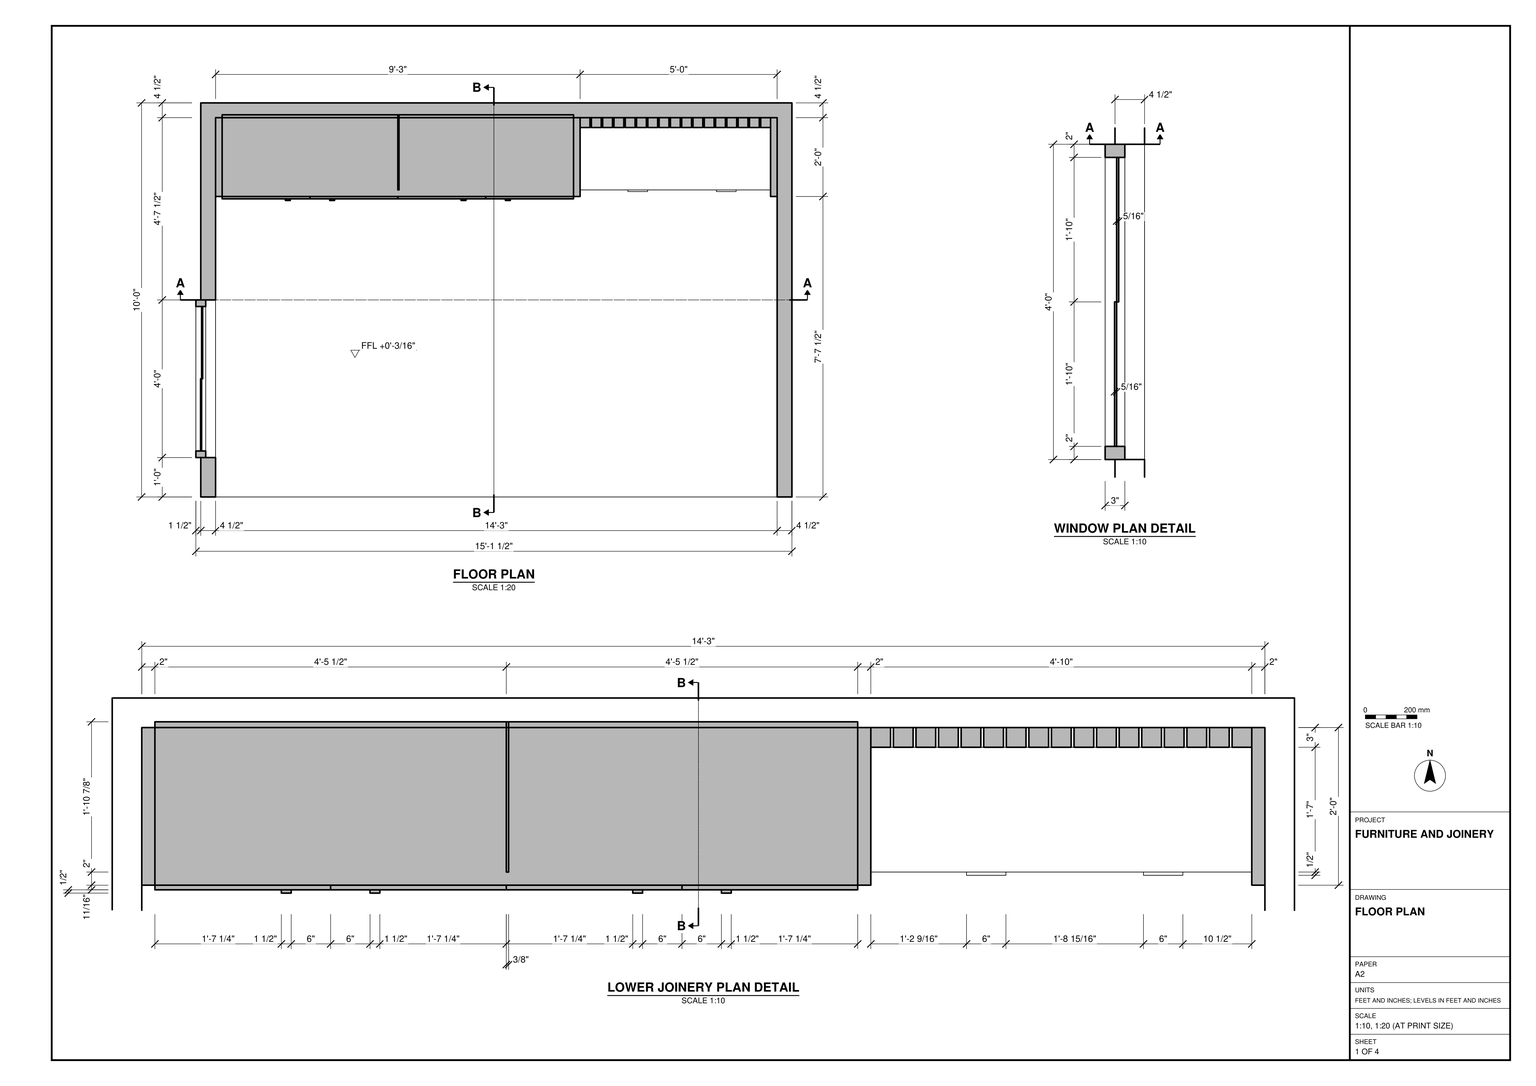
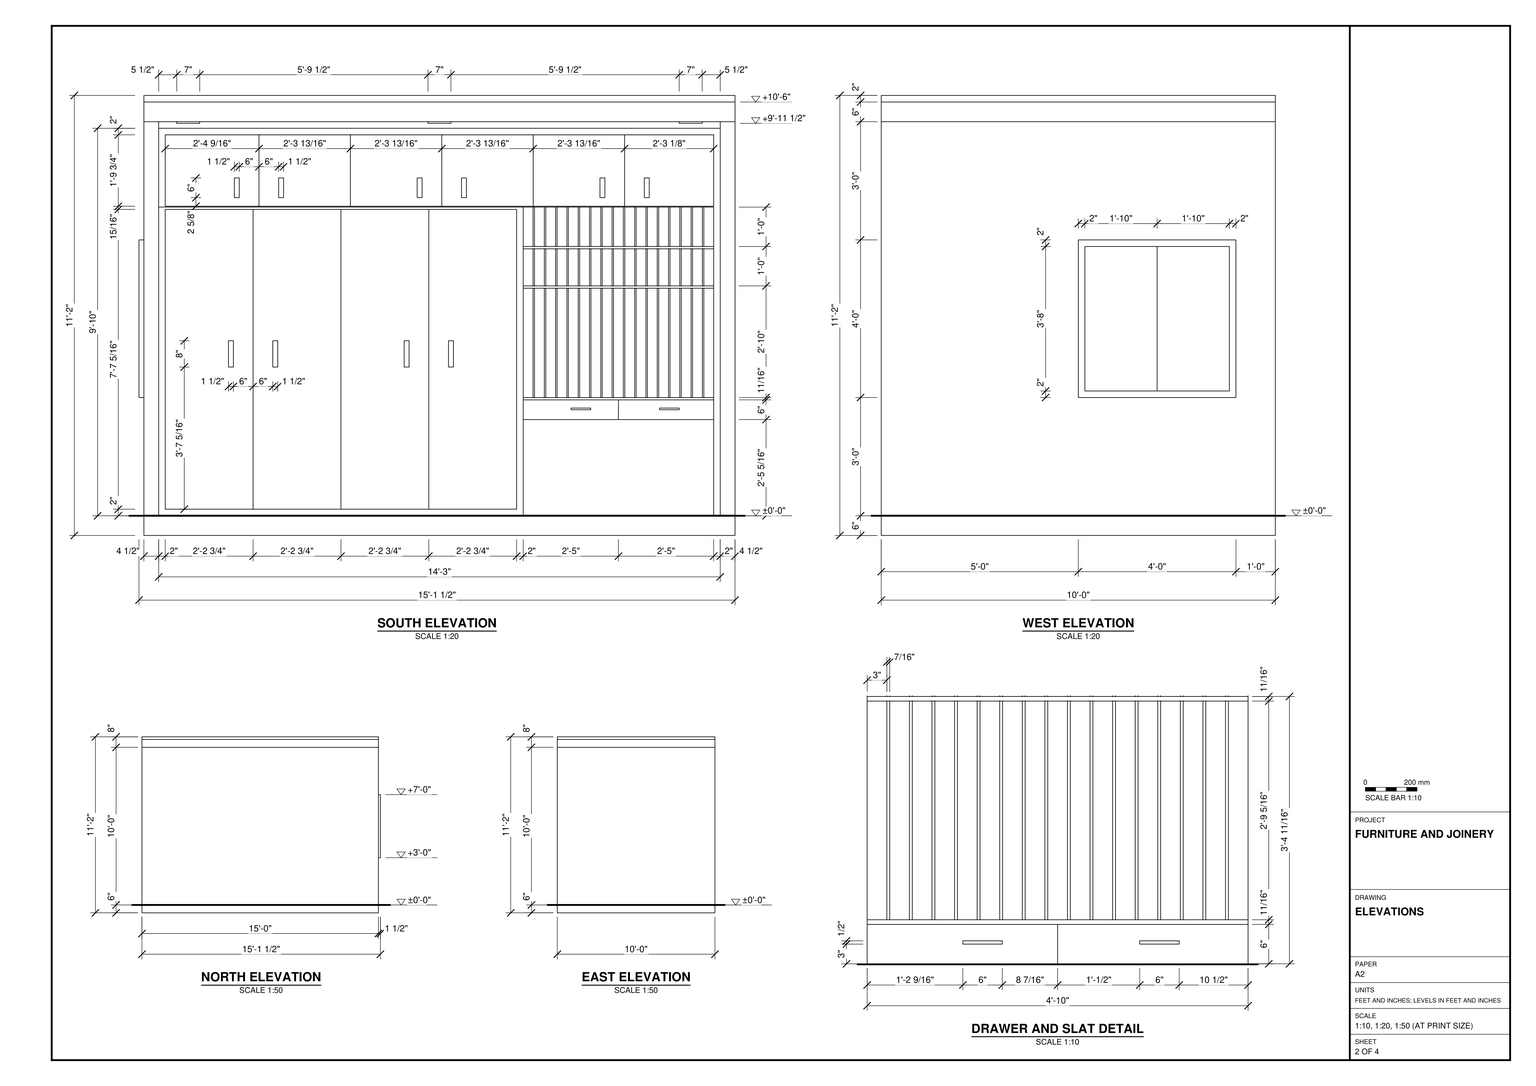
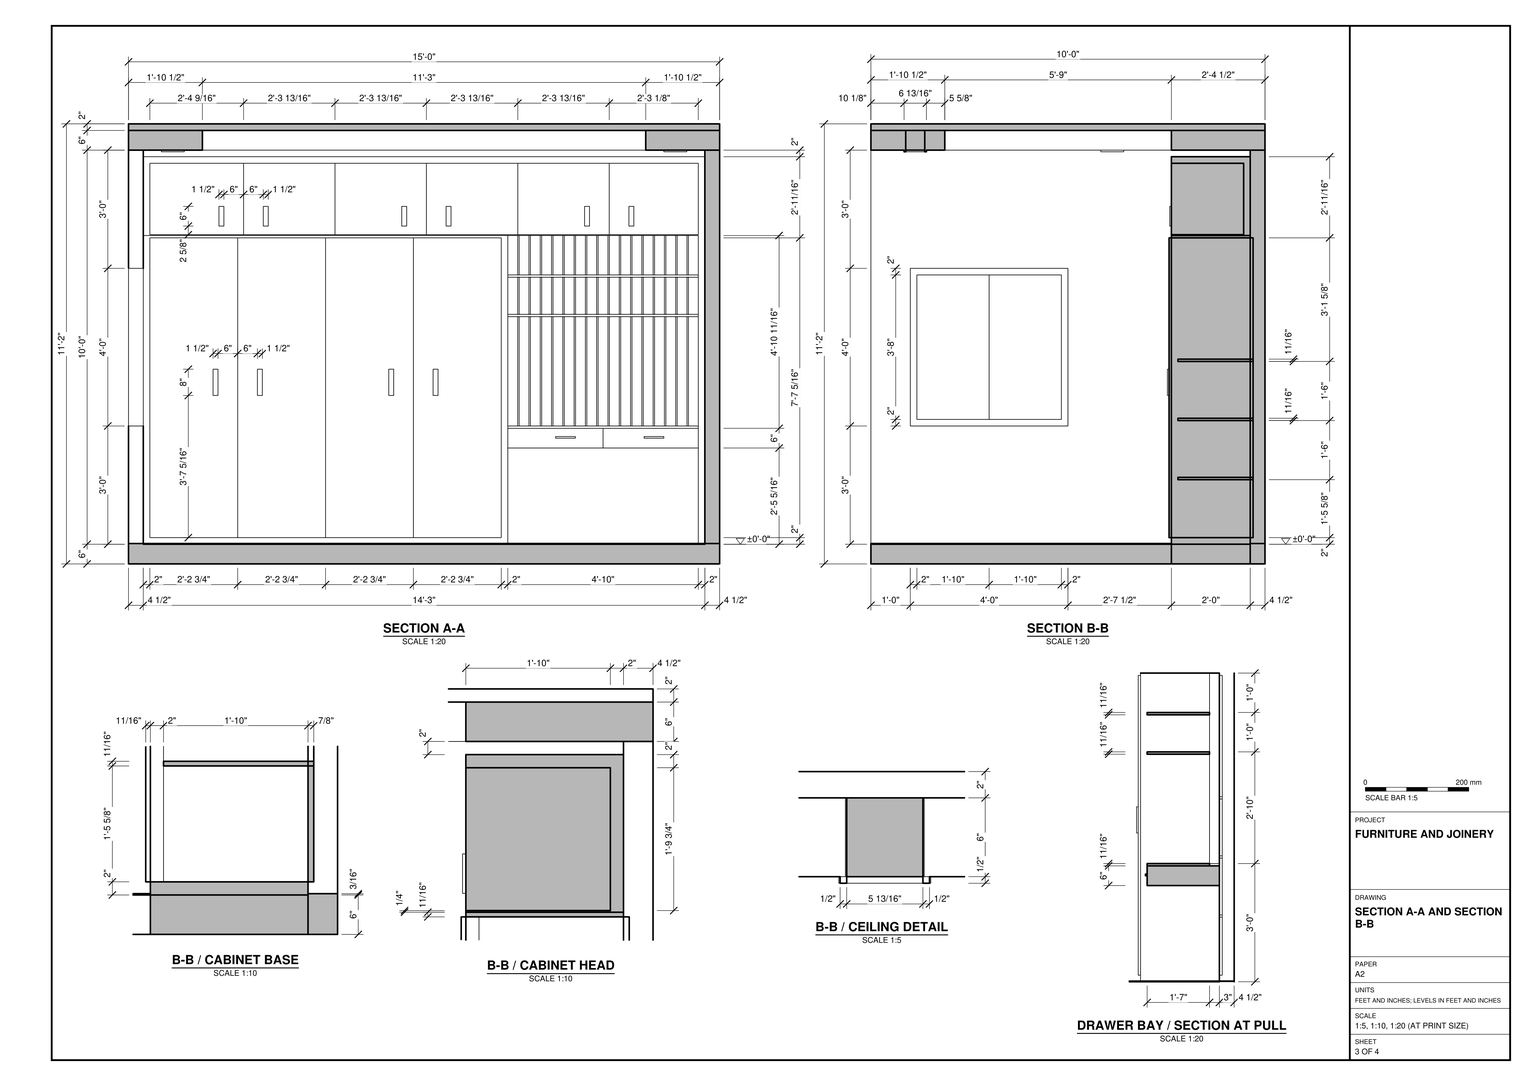
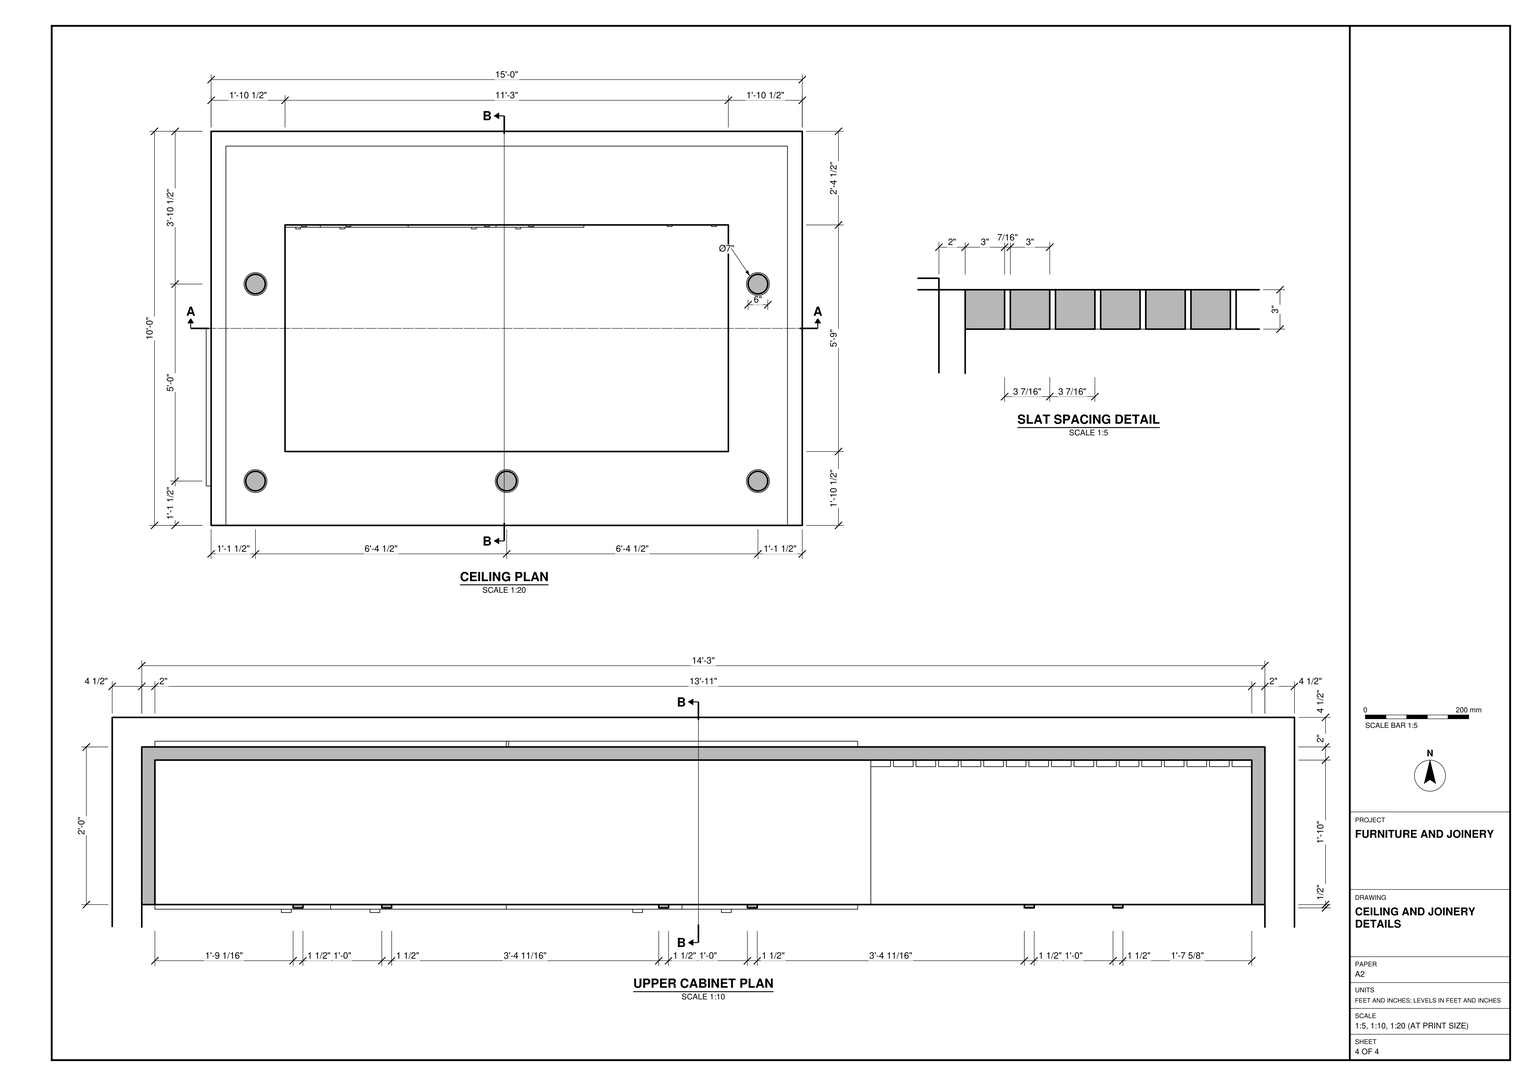
Build the wall-to-wall storage unit and its surrounding room shell in SketchUp using task_files/diagram_01.pdf. Work in feet and inches. The overall model is 15'-1 1/2" wide, 10'-0" deep and 11'-2" high. Use ±0'-0" as the ground-floor datum.

Model the floor slab, the 4 1/2" back and side walls, and the ceiling slab with its deeper perimeter section. Leave the front open as shown in plan. Fit the framed, two-panel window into the west wall at the position shown in the west elevation.

Run the joinery along the back wall. Facing the unit, place the tall wardrobe on the left, with its plinth, internal partition, shelves and paired door fronts. Continue the overhead cupboards across both the wardrobe and the open bay on the right. In that bay, model the vertical slats behind the shelves and the two shallow drawers side by side, leaving clear space beneath them. Follow the elevations for the size and orientation of the pulls.

Keep shell elements and individual joinery pieces in separate groups or components, and use components for repeated parts. Any decor or loose items may be suitable library components. Save one SketchUp model as output_files/built_in_wardrobe_with_a_slatted_drawer_bay.skp.

# SketchUp Ruby script. Lengths in inches.
U = 1.inch
M = Sketchup.active_model
def pt(a) = Geom::Point3d.new(a.map { |v| v * U })
def face(e, loops, mat)
  f = e.add_face(loops[0].map { |a| pt(a) })
  loops[1..].each { |l| e.add_face(l.map { |a| pt(a) }).erase! }
  f.material = f.back_material = mat if mat
  f
end
# faces: each face lists its corners as indices into pts; further lists are holes
def faces(e, pts, list, mat = nil) = list.each { |f| face(e, (f[0].is_a?(Array) ? f : [f]).map { |l| l.map { |i| pts[i] } }, mat) }
# xy, xz, yz: faces in a plane at the given z, y or x. An outline is a flat list of corners, or four numbers for a rectangle; further outlines are holes
def ring(l) = l.size == 4 ? [[l[0], l[1]], [l[2], l[1]], [l[2], l[3]], [l[0], l[3]]] : l.each_slice(2).to_a
def flat(e, list, mat, &to3) = list.each { |f| face(e, (f[0].is_a?(Array) ? f : [f]).map { |l| ring(l).map { |u, v| to3.(u, v) } }, mat) }
def xy(e, z, list, mat = nil) = flat(e, list, mat) { |x, y| [x, y, z] }
def xz(e, y, list, mat = nil) = flat(e, list, mat) { |x, z| [x, y, z] }
def yz(e, x, list, mat = nil) = flat(e, list, mat) { |y, z| [x, y, z] }
def lines(e, pts, list) = list.each { |a, b| e.add_line(pt(pts[a]), pt(pts[b])) }
# prism: a flat outline (further loops are holes) pulled along v
def prism(e, loops, v, mat = nil)
  f = face(e, loops, mat); d = Geom::Vector3d.new(v.map { |x| x * U })
  f.pushpull(f.normal.samedirection?(d) ? d.length : -d.length)
end
def box(e, o, s, mat = nil) = prism(e, [[o, [o[0] + s[0], o[1], o[2]], [o[0] + s[0], o[1] + s[1], o[2]], [o[0], o[1] + s[1], o[2]]]], [0, 0, s[2]], mat)
def at(x, y, z, deg = 0) = Geom::Transformation.translation(pt([x, y, z])) * Geom::Transformation.rotation(ORIGIN, Z_AXIS, deg.degrees)
def axes(o, x, y, z) = Geom::Transformation.new([*x, 0, *y, 0, *z, 0, *pt(o).to_a, 1])
def part(name) = M.definitions.add(name)
# library, detail: a bought-in or finely detailed component or shape, given as its bounding box
def library(name, o, s) = part(name).tap { |d| box(d.entities, o, s) }
def detail(e, o, s) = box(e.add_group.entities, o, s)
def put(e, d, t, mat = nil) = e.add_instance(d, t).tap { |i| i.material = mat if mat }
def group(e, t, mat = nil) = e.add_group.tap { |g| g.transformation = t; g.material = mat if mat }.entities
root = M.entities
M.materials.add("Carpaint Stochastic Gold").color = [216, 180, 130]
M.materials.add("Flooring Parquet Parallel E01 120cm").color = [119, 88, 63]
M.materials.add("Glass Yellow 001").color = [0, 0, 0]
M.materials["Glass Yellow 001"].alpha = 0.1
M.materials.add("Marble Black 100cm").color = [32, 32, 32]
M.materials.add("Metal Sandblasted Black 200cm").color = [86, 90, 95]
M.materials.add("Wood Tiles Dark Shiny 02 100cm").color = [42, 30, 20]
M.materials.add("[0023_FireBrick]").color = [236, 223, 216]
M.materials.add("[Color C06]").color = [166, 138, 92]
M.materials.add("[Color D01]").color = [255, 242, 204]
M.materials.add("[Color D05]").color = [234, 208, 139]
M.materials.add("[Color D06]").color = [170, 123, 68]
M.materials.add("[Color M00]").color = [255, 255, 255]
M.materials.add("[Color M04]").color = [142, 142, 142]
M.materials.add("[Color M06]").color = [86, 86, 86]
c1 = part("Group\#25")
box(c1.entities,[0,0,0],[0.31,22,44])
c2 = part("Group\#2")
box(c2.entities,[0,2,-0.35],[107,22.875,0.7])
p = [[24,22.5,126],[24,91.5,126],[159,91.5,126],[159,22.5,126]]
lines(root,p,[[0,1],[1,2],[2,3],[3,0]])
g1 = group(root,at(1.5,0,0))
xy(g1,0,[[4.5,0,175.5,115.5]],"[Color M04]")
xy(g1,36,[[0,12,4.5,60]],"[Color M04]")
xy(g1,84,[[0,12,4.5,60]],"[Color M04]")
xy(g1,120,[[0,0,4.5,0,4.5,115.5,175.5,115.5,175.5,0,180,0,180,120,0,120]],"[Color M04]")
xz(g1,0,[[0,0,4.5,120],[175.5,0,180,120]],"[Color M04]")
xz(g1,12,[[0,36,4.5,84]],"[Color M04]")
xz(g1,60,[[0,36,4.5,84]],"[Color M04]")
xz(g1,115.5,[[4.5,0,175.5,120]],"[Color M04]")
xz(g1,120,[[0,0,180,120]],"[Color M04]")
yz(g1,0,[[[0,0,120,120],[12,36,60,84]]],"[Color M04]")
yz(g1,4.5,[[[0,0,115.5,120],[12,36,60,84]]],"[Color M04]")
yz(g1,175.5,[[0,0,115.5,120]],"[Color M04]")
yz(g1,180,[[0,0,120,120]],"[Color M04]")
g2 = group(g1,at(0,12,36))
prism(g2,[[[-1.5,48,0],[-1.5,0,0],[-1.5,0,48],[-1.5,48,48]],[[-1.5,46,2],[-1.5,46,46],[-1.5,2,46],[-1.5,2,2]]],[3,0,0],"Metal Sandblasted Black 200cm")
put(g1,c1,at(0.25,36,38),"Glass Yellow 001")
put(g1,c1,at(-0.06,14,38),"Glass Yellow 001")
put(root,c2,at(8,91.5,20))
put(root,c2,at(8,91.5,38))
put(root,c2,at(8,91.5,56))
g3 = group(root,at(61.5,91.5,2.71))
prism(g3,[[[0,2,-0.71],[0,2,90.58],[0,24,90.58],[0,24.875,90.58],[0,24.875,89.875],[0,24.875,17.29],[0,24.875,16.58],[0,24.875,-0.71]]],[0.35,0,0])
g4 = group(root,at(8,91.5,2),"[0023_FireBrick]")
box(g4,[0,-0.71,0],[26.75,0.71,91.29],"[Color C06]")
g5 = group(root,at(34.75,91.5,2),"[Color D06]")
box(g5,[0,-0.71,0],[26.75,0.71,91.29],"[Color C06]")
g6 = group(root,at(61.5,91.5,2),"[Color M06]")
box(g6,[0,-0.71,0],[26.75,0.71,91.29],"[Color C06]")
g7 = group(root,at(88.25,91.5,2),"[Color M06]")
box(g7,[0,-0.71,0],[26.75,0.71,91.29],"[Color C06]")
g8 = group(root,at(6,115.5,94))
xy(g8,-94,[[169,-24,171,0]])
xy(g8,0,[[0,-24,169,0]],"Flooring Parquet Parallel E01 120cm")
xy(g8,0.25,[[2,-24,169,-2]])
xy(g8,22,[[2,-24,169,-2]])
xy(g8,24,[[0,-24,171,0]])
xz(g8,-24,[[[169,-94,171,-94,171,24,0,24,0,0,169,0],[2,0.25,169,22]]],"Flooring Parquet Parallel E01 120cm")
xz(g8,-24,[[2,0.25,30.54,22],[30.54,0.25,58.375,22],[58.375,0.25,86.21,22],[86.21,0.25,114.04,22],[114.04,0.25,141.875,22],
  [141.875,0.25,169,22]],"[Color C06]")
xz(g8,-2,[[2,0.25,169,22]])
xz(g8,0,[[169,-94,169,0,0,0,0,24,171,24,171,-94]])
yz(g8,0,[[-24,0,0,24]])
yz(g8,2,[[-24,0.25,-2,22]])
yz(g8,169,[[-24,0.25,-2,22]])
yz(g8,169,[[-24,-94,0,0]],"Flooring Parquet Parallel E01 120cm")
yz(g8,171,[[-24,-94,0,24]])
g9 = group(root,at(117,113.03,36),"Wood Tiles Dark Shiny 02 100cm")
box(g9,[0,-0.53,0],[3,3,58],"Wood Tiles Dark Shiny 02 100cm")
g10 = group(root,at(120.4375,113.03,36),"Wood Tiles Dark Shiny 02 100cm")
box(g10,[0,-0.53,0],[3,3,58],"Wood Tiles Dark Shiny 02 100cm")
g11 = group(root,at(123.875,113.03,36),"Wood Tiles Dark Shiny 02 100cm")
box(g11,[0,-0.53,0],[3,3,58],"Wood Tiles Dark Shiny 02 100cm")
g12 = group(root,at(127.3125,113.03,36),"Wood Tiles Dark Shiny 02 100cm")
box(g12,[0,-0.53,0],[3,3,58],"Wood Tiles Dark Shiny 02 100cm")
g13 = group(root,at(130.75,113.03,36),"Wood Tiles Dark Shiny 02 100cm")
box(g13,[0,-0.53,0],[3,3,58],"Wood Tiles Dark Shiny 02 100cm")
g14 = group(root,at(134.1875,113.03,36),"Wood Tiles Dark Shiny 02 100cm")
box(g14,[0,-0.53,0],[3,3,58],"Wood Tiles Dark Shiny 02 100cm")
g15 = group(root,at(137.625,113.03,36),"Wood Tiles Dark Shiny 02 100cm")
box(g15,[0,-0.53,0],[3,3,58],"Wood Tiles Dark Shiny 02 100cm")
g16 = group(root,at(141.0625,113.03,36),"Wood Tiles Dark Shiny 02 100cm")
box(g16,[0,-0.53,0],[3,3,58],"Wood Tiles Dark Shiny 02 100cm")
g17 = group(root,at(144.5,113.03,36),"Wood Tiles Dark Shiny 02 100cm")
box(g17,[0,-0.53,0],[3,3,58],"Wood Tiles Dark Shiny 02 100cm")
g18 = group(root,at(147.9375,113.03,36),"Wood Tiles Dark Shiny 02 100cm")
box(g18,[0,-0.53,0],[3,3,58],"Wood Tiles Dark Shiny 02 100cm")
g19 = group(root,at(151.375,113.03,36),"Wood Tiles Dark Shiny 02 100cm")
box(g19,[0,-0.53,0],[3,3,58],"Wood Tiles Dark Shiny 02 100cm")
g20 = group(root,at(154.8125,113.03,36),"Wood Tiles Dark Shiny 02 100cm")
box(g20,[0,-0.53,0],[3,3,58],"Wood Tiles Dark Shiny 02 100cm")
g21 = group(root,at(158.25,113.03,36),"Wood Tiles Dark Shiny 02 100cm")
box(g21,[0,-0.53,0],[3,3,58],"Wood Tiles Dark Shiny 02 100cm")
g22 = group(root,at(161.6875,113.03,36),"Wood Tiles Dark Shiny 02 100cm")
box(g22,[0,-0.53,0],[3,3,58],"Wood Tiles Dark Shiny 02 100cm")
g23 = group(root,at(165.125,113.03,36),"Wood Tiles Dark Shiny 02 100cm")
box(g23,[0,-0.53,0],[3,3,58],"Wood Tiles Dark Shiny 02 100cm")
g24 = group(root,at(168.5625,113.03,36),"Wood Tiles Dark Shiny 02 100cm")
box(g24,[0,-0.53,0],[3,3,58],"Wood Tiles Dark Shiny 02 100cm")
g25 = group(root,at(172,113.03,36),"Wood Tiles Dark Shiny 02 100cm")
box(g25,[0,-0.53,0],[3,3,58],"Wood Tiles Dark Shiny 02 100cm")
g26 = group(root,at(117,112.5,81.29),"Flooring Parquet Parallel E01 120cm")
box(g26,[0,-19,0],[58,19,0.71],"Flooring Parquet Parallel E01 120cm")
g27 = group(root,at(117,112.5,69.29),"Flooring Parquet Parallel E01 120cm")
box(g27,[0,-19,0],[58,19,0.71],"Flooring Parquet Parallel E01 120cm")
g28 = group(root,at(117,112.5,35.29),"Flooring Parquet Parallel E01 120cm")
box(g28,[0,-19,0],[58,19,0.71],"Flooring Parquet Parallel E01 120cm")
g29 = group(root,at(117,115.5,29.29))
prism(g29,[[[0,0,0],[58,0,0],[58,-22,0],[29,-22,0],[0,-22,0]]],[0,0,6],"Flooring Parquet Parallel E01 120cm")
g30 = group(g29,at(14.57,-22,2.5),"[Color D05]")
box(g30,[0,-0.5,0.5],[6,0.5,0.5])
g31 = group(g29,at(41.51,-22,2.5),"[Color D05]")
box(g31,[0,-0.5,0.5],[6,0.5,0.5])
g32 = group(root,at(1.5,0,0))
xy(g32,-6,[[[0,0,180,120],[4.5,91.5,115.5,115.5]],[4.5,91.5,115.5,115.5]])
xy(g32,0.2,[[[0,0,180,120],[4.5,91.5,115.5,115.5]]],"Marble Black 100cm")
xy(g32,2,[[6.5,91.5,113.5,116.375]])
xy(g32,93.29,[[6.5,91.5,113.5,116.375]])
xy(g32,94,[[4.5,91.5,115.5,115.5]])
xz(g32,0,[[0,-6,180,0.2]])
xz(g32,91.5,[[4.5,-6,115.5,0.2]])
xz(g32,91.5,[[[4.5,0.2,115.5,94],[6.5,2,113.5,93.29]]],"Flooring Parquet Parallel E01 120cm")
xz(g32,115.5,[[4.5,-6,115.5,0.2]])
xz(g32,116.375,[[6.5,2,113.5,20],[6.5,20,60,93.29],[60,20,113.5,93.29]])
xz(g32,120,[[0,-6,180,0.2]])
yz(g32,0,[[0,-6,120,0.2]])
yz(g32,4.5,[[91.5,-6,115.5,0.2],[91.5,0.2,115.5,94]])
yz(g32,6.5,[[91.5,2,116.375,93.29]])
yz(g32,113.5,[[91.5,2,116.375,93.29]])
yz(g32,115.5,[[91.5,-6,115.5,0.2]])
yz(g32,115.5,[[91.5,0.2,115.5,94]],"[Color C06]")
yz(g32,180,[[0,-6,120,0.2]])
g33 = group(root,at(29.04,91.5,96.875),"[Color D05]")
box(g33,[0,-0.5,0],[1.5,0.5,6],"[Color D05]")
g34 = group(root,at(42.54,91.5,96.875),"Carpaint Stochastic Gold")
box(g34,[0,-0.5,0],[1.5,0.5,6],"[Color D05]")
g35 = group(root,at(84.71,91.5,96.875),"Carpaint Stochastic Gold")
xy(g35,0,[[0,-0.5,1.5,0]],"Metal Sandblasted Black 200cm")
xy(g35,6,[[0,-0.5,1.5,0]],"Metal Sandblasted Black 200cm")
xz(g35,-0.5,[[0,0,1.5,6]],"[Color D05]")
xz(g35,0,[[0,0,1.5,6]],"Metal Sandblasted Black 200cm")
yz(g35,0,[[-0.5,0,0,6]],"Metal Sandblasted Black 200cm")
yz(g35,1.5,[[-0.5,0,0,6]],"Metal Sandblasted Black 200cm")
g36 = group(root,at(98.21,91.5,96.875),"Carpaint Stochastic Gold")
box(g36,[0,-0.5,0],[1.5,0.5,6],"[Color D05]")
g37 = group(root,at(140.375,91.5,96.875),"Carpaint Stochastic Gold")
box(g37,[0,-0.5,0],[1.5,0.5,6],"[Color D05]")
g38 = group(root,at(153.875,91.5,96.875),"[Color D05]")
box(g38,[0,-0.5,0],[1.5,0.5,6],"[Color D05]")
g39 = group(root,at(27.25,90.79,45.29),"Carpaint Stochastic Gold")
box(g39,[0,-0.5,0],[1.5,0.5,8],"[Color D05]")
g40 = group(root,at(40.75,90.79,45.29),"Carpaint Stochastic Gold")
box(g40,[0,-0.5,0],[1.5,0.5,8],"[Color D05]")
g41 = group(root,at(80.75,90.79,45.29),"Metal Sandblasted Black 200cm")
box(g41,[0,-0.5,0],[1.5,0.5,8],"[Color D05]")
g42 = group(root,at(94.25,90.79,45.29),"Carpaint Stochastic Gold")
box(g42,[0,-0.5,0],[1.5,0.5,8],"[Color D05]")
g43 = group(root,at(1.5,0,120))
xy(g43,-0.5,[[[13.5,10,12.59,10.12,11.75,10.47,11.03,11.03,10.47,11.75,10.12,12.59,10,13.5,10.12,14.41,10.47,15.25,11.03,15.97,11.75,16.53,12.59,16.88,13.5,17,14.41,16.88,15.25,16.53,15.97,15.97,16.53,15.25,16.88,14.41,17,13.5,16.88,12.59,16.53,11.75,15.97,11.03,15.25,10.47,14.41,10.12],[13.5,10.5,14.28,10.6,15,10.9,15.62,11.38,16.1,12,16.4,12.72,16.5,13.5,16.4,14.28,16.1,15,15.62,15.62,15,16.1,14.28,16.4,13.5,16.5,12.72,16.4,12,16.1,11.38,15.62,10.9,15,10.6,14.28,10.5,13.5,10.6,12.72,10.9,12,11.38,11.38,12,10.9,12.72,10.6]],[[90,10,89.09,10.12,88.25,10.47,87.53,11.03,86.97,11.75,86.62,12.59,86.5,13.5,86.62,14.41,86.97,15.25,87.53,15.97,88.25,16.53,89.09,16.88,90,17,90.91,16.88,91.75,16.53,92.47,15.97,93.03,15.25,93.38,14.41,93.5,13.5,93.38,12.59,93.03,11.75,92.47,11.03,91.75,10.47,90.91,10.12],[90,10.5,90.78,10.6,91.5,10.9,92.12,11.38,92.6,12,92.9,12.72,93,13.5,92.9,14.28,92.6,15,92.12,15.62,91.5,16.1,90.78,16.4,90,16.5,89.22,16.4,88.5,16.1,87.88,15.62,87.4,15,87.1,14.28,87,13.5,87.1,12.72,87.4,12,87.88,11.38,88.5,10.9,89.22,10.6]],[[166.5,10,165.59,10.12,164.75,10.47,164.03,11.03,163.47,11.75,163.12,12.59,163,13.5,163.12,14.41,163.47,15.25,164.03,15.97,164.75,16.53,165.59,16.88,166.5,17,167.41,16.88,168.25,16.53,168.97,15.97,169.53,15.25,169.88,14.41,170,13.5,169.88,12.59,169.53,11.75,168.97,11.03,168.25,10.47,167.41,10.12],[166.5,10.5,167.28,10.6,168,10.9,168.62,11.38,169.1,12,169.4,12.72,169.5,13.5,169.4,14.28,169.1,15,168.62,15.62,168,16.1,167.28,16.4,166.5,16.5,165.72,16.4,165,16.1,164.38,15.62,163.9,15,163.6,14.28,163.5,13.5,163.6,12.72,163.9,12,164.38,11.38,165,10.9,165.72,10.6]],[[166.47,70,165.57,70.125,164.73,70.48,164.01,71.04,163.46,71.77,163.11,72.62,163,73.53,163.125,74.43,163.48,75.27,164.04,75.99,164.77,76.54,165.62,76.89,166.53,77,167.43,76.875,168.27,76.52,168.99,75.96,169.54,75.23,169.89,74.38,170,73.47,169.875,72.57,169.52,71.73,168.96,71.01,168.23,70.46,167.38,70.11],[166.48,70.5,167.25,70.6,167.98,70.89,168.61,71.36,169.09,71.98,169.39,72.7,169.5,73.48,169.4,74.25,169.11,74.98,168.64,75.61,168.02,76.09,167.3,76.39,166.52,76.5,165.75,76.4,165.02,76.11,164.39,75.64,163.91,75.02,163.61,74.3,163.5,73.52,163.6,72.75,163.89,72.02,164.36,71.39,164.98,70.91,165.7,70.61]],[[13.2,70.01,12.3125,70.21,11.5,70.63,10.82,71.24,10.33,72.01,10.05,72.88,10.01,73.8,10.21,74.6875,10.63,75.5,11.24,76.18,12.01,76.67,12.88,76.95,13.8,76.99,14.6875,76.79,15.5,76.37,16.18,75.76,16.67,74.99,16.95,74.12,16.99,73.2,16.79,72.3125,16.37,71.5,15.76,70.82,14.99,70.33,14.12,70.05],[13.25,70.51,14.03,70.55,14.77,70.78,15.43,71.21,15.96,71.79,16.32,72.48,16.49,73.25,16.45,74.03,16.22,74.77,15.79,75.43,15.21,75.96,14.52,76.32,13.75,76.49,12.97,76.45,12.23,76.22,11.57,75.79,11.04,75.21,10.68,74.52,10.51,73.75,10.55,72.97,10.78,72.23,11.21,71.57,11.79,71.04,12.48,70.68]]],"[Color M00]")
xy(g43,0,[[[0,0,180,120],[22.5,22.5,157.5,91.5],[13.5,10,14.41,10.12,15.25,10.47,15.97,11.03,16.53,11.75,16.88,12.59,17,13.5,16.88,14.41,16.53,15.25,15.97,15.97,15.25,16.53,14.41,16.88,13.5,17,12.59,16.88,11.75,16.53,11.03,15.97,10.47,15.25,10.12,14.41,10,13.5,10.12,12.59,10.47,11.75,11.03,11.03,11.75,10.47,12.59,10.12],[166.5,10,167.41,10.12,168.25,10.47,168.97,11.03,169.53,11.75,169.88,12.59,170,13.5,169.88,14.41,169.53,15.25,168.97,15.97,168.25,16.53,167.41,16.88,166.5,17,165.59,16.88,164.75,16.53,164.03,15.97,163.47,15.25,163.12,14.41,163,13.5,163.12,12.59,163.47,11.75,164.03,11.03,164.75,10.47,165.59,10.12],[90,10,90.91,10.12,91.75,10.47,92.47,11.03,93.03,11.75,93.38,12.59,93.5,13.5,93.38,14.41,93.03,15.25,92.47,15.97,91.75,16.53,90.91,16.88,90,17,89.09,16.88,88.25,16.53,87.53,15.97,86.97,15.25,86.62,14.41,86.5,13.5,86.62,12.59,86.97,11.75,87.53,11.03,88.25,10.47,89.09,10.12],[13.2,70.01,14.12,70.05,14.99,70.33,15.76,70.82,16.37,71.5,16.79,72.3125,16.99,73.2,16.95,74.12,16.67,74.99,16.18,75.76,15.5,76.37,14.6875,76.79,13.8,76.99,12.88,76.95,12.01,76.67,11.24,76.18,10.63,75.5,10.21,74.6875,10.01,73.8,10.05,72.88,10.33,72.01,10.82,71.24,11.5,70.63,12.3125,70.21],[166.47,70,167.38,70.11,168.23,70.46,168.96,71.01,169.52,71.73,169.875,72.57,170,73.47,169.89,74.38,169.54,75.23,168.99,75.96,168.27,76.52,167.43,76.875,166.53,77,165.62,76.89,164.77,76.54,164.04,75.99,163.48,75.27,163.125,74.43,163,73.53,163.11,72.62,163.46,71.77,164.01,71.04,164.73,70.48,165.57,70.125]]],"[Color D01]")
xy(g43,0,[[13.5,10.5,12.72,10.6,12,10.9,11.38,11.38,10.9,12,10.6,12.72,10.5,13.5,10.6,14.28,10.9,15,11.38,15.62,12,16.1,12.72,16.4,13.5,16.5,14.28,16.4,15,16.1,15.62,15.62,16.1,15,16.4,14.28,16.5,13.5,16.4,12.72,16.1,12,15.62,11.38,15,10.9,14.28,10.6],[90,10.5,89.22,10.6,88.5,10.9,87.88,11.38,87.4,12,87.1,12.72,87,13.5,87.1,14.28,87.4,15,87.88,15.62,88.5,16.1,89.22,16.4,90,16.5,90.78,16.4,91.5,16.1,92.12,15.62,92.6,15,92.9,14.28,93,13.5,92.9,12.72,92.6,12,92.12,11.38,91.5,10.9,90.78,10.6],[166.5,10.5,165.72,10.6,165,10.9,164.38,11.38,163.9,12,163.6,12.72,163.5,13.5,163.6,14.28,163.9,15,164.38,15.62,165,16.1,165.72,16.4,166.5,16.5,167.28,16.4,168,16.1,168.62,15.62,169.1,15,169.4,14.28,169.5,13.5,169.4,12.72,169.1,12,168.62,11.38,168,10.9,167.28,10.6],[166.48,70.5,165.7,70.61,164.98,70.91,164.36,71.39,163.89,72.02,163.6,72.75,163.5,73.52,163.61,74.3,163.91,75.02,164.39,75.64,165.02,76.11,165.75,76.4,166.52,76.5,167.3,76.39,168.02,76.09,168.64,75.61,169.11,74.98,169.4,74.25,169.5,73.48,169.39,72.7,169.09,71.98,168.61,71.36,167.98,70.89,167.25,70.6],[13.25,70.51,12.48,70.68,11.79,71.04,11.21,71.57,10.78,72.23,10.55,72.97,10.51,73.75,10.68,74.52,11.04,75.21,11.57,75.79,12.23,76.22,12.97,76.45,13.75,76.49,14.52,76.32,15.21,75.96,15.79,75.43,16.22,74.77,16.45,74.03,16.49,73.25,16.32,72.48,15.96,71.79,15.43,71.21,14.77,70.78,14.03,70.55]],"[Color D05]")
xy(g43,6,[[[0,0,180,120],[4.5,4.5,175.5,115.5]],[[4.5,4.5,175.5,115.5],[22.5,22.5,157.5,91.5],[166.48,70.5,165.7,70.61,164.98,70.91,164.36,71.39,163.89,72.02,163.6,72.75,163.5,73.52,163.61,74.3,163.91,75.02,164.39,75.64,165.02,76.11,165.75,76.4,166.52,76.5,167.3,76.39,168.02,76.09,168.64,75.61,169.11,74.98,169.4,74.25,169.5,73.48,169.39,72.7,169.09,71.98,168.61,71.36,167.98,70.89,167.25,70.6],[13.5,10.5,12.72,10.6,12,10.9,11.38,11.38,10.9,12,10.6,12.72,10.5,13.5,10.6,14.28,10.9,15,11.38,15.62,12,16.1,12.72,16.4,13.5,16.5,14.28,16.4,15,16.1,15.62,15.62,16.1,15,16.4,14.28,16.5,13.5,16.4,12.72,16.1,12,15.62,11.38,15,10.9,14.28,10.6],[166.5,10.5,165.72,10.6,165,10.9,164.38,11.38,163.9,12,163.6,12.72,163.5,13.5,163.6,14.28,163.9,15,164.38,15.62,165,16.1,165.72,16.4,166.5,16.5,167.28,16.4,168,16.1,168.62,15.62,169.1,15,169.4,14.28,169.5,13.5,169.4,12.72,169.1,12,168.62,11.38,168,10.9,167.28,10.6],[13.25,70.51,12.48,70.68,11.79,71.04,11.21,71.57,10.78,72.23,10.55,72.97,10.51,73.75,10.68,74.52,11.04,75.21,11.57,75.79,12.23,76.22,12.97,76.45,13.75,76.49,14.52,76.32,15.21,75.96,15.79,75.43,16.22,74.77,16.45,74.03,16.49,73.25,16.32,72.48,15.96,71.79,15.43,71.21,14.77,70.78,14.03,70.55],[90,10.5,89.22,10.6,88.5,10.9,87.88,11.38,87.4,12,87.1,12.72,87,13.5,87.1,14.28,87.4,15,87.88,15.62,88.5,16.1,89.22,16.4,90,16.5,90.78,16.4,91.5,16.1,92.12,15.62,92.6,15,92.9,14.28,93,13.5,92.9,12.72,92.6,12,92.12,11.38,91.5,10.9,90.78,10.6]]],"[Color M00]")
xz(g43,0,[[0,0,180,6]],"[Color M00]")
xz(g43,22.5,[[22.5,0,157.5,6]],"[Color M00]")
xz(g43,91.5,[[22.5,0,157.5,6]],"[Color D01]")
xz(g43,120,[[0,0,180,6]],"[Color M00]")
yz(g43,0,[[0,0,120,6]],"[Color M00]")
yz(g43,22.5,[[22.5,0,91.5,6]],"[Color D01]")
yz(g43,157.5,[[22.5,0,91.5,6]],"[Color D01]")
yz(g43,180,[[0,0,120,6]],"[Color M00]")
p = [[13.5,10,0],[12.59,10.12,0],[12.59,10.12,-0.5],[13.5,10,-0.5],[14.41,10.12,0],[14.41,10.12,-0.5],
  [90,10,0],[89.09,10.12,0],[89.09,10.12,-0.5],[90,10,-0.5],[90.91,10.12,0],[90.91,10.12,-0.5],
  [166.5,10,0],[165.59,10.12,0],[165.59,10.12,-0.5],[166.5,10,-0.5],[167.41,10.12,0],[167.41,10.12,-0.5],
  [11.75,10.47,0],[11.75,10.47,-0.5],[15.25,10.47,0],[15.25,10.47,-0.5],[88.25,10.47,0],[88.25,10.47,-0.5],
  [91.75,10.47,0],[91.75,10.47,-0.5],[164.75,10.47,0],[164.75,10.47,-0.5],[168.25,10.47,0],[168.25,10.47,-0.5],
  [11.03,11.03,0],[11.03,11.03,-0.5],[12.72,10.6,0],[13.5,10.5,0],[13.5,10.5,-0.5],[12.72,10.6,-0.5],
  [14.28,10.6,0],[14.28,10.6,-0.5],[15.97,11.03,0],[15.97,11.03,-0.5],[87.53,11.03,0],[87.53,11.03,-0.5],
  [89.22,10.6,0],[90,10.5,0],[90,10.5,-0.5],[89.22,10.6,-0.5],[90.78,10.6,0],[90.78,10.6,-0.5],
  [92.47,11.03,0],[92.47,11.03,-0.5],[164.03,11.03,0],[164.03,11.03,-0.5],[165.72,10.6,0],[166.5,10.5,0],
  [166.5,10.5,-0.5],[165.72,10.6,-0.5],[167.28,10.6,0],[167.28,10.6,-0.5],[168.97,11.03,0],[168.97,11.03,-0.5],
  [12,10.9,0],[12,10.9,-0.5],[15,10.9,0],[15,10.9,-0.5],[88.5,10.9,0],[88.5,10.9,-0.5],
  [91.5,10.9,0],[91.5,10.9,-0.5],[165,10.9,0],[165,10.9,-0.5],[168,10.9,0],[168,10.9,-0.5],
  [11.38,11.38,0],[11.38,11.38,-0.5],[15.62,11.38,0],[15.62,11.38,-0.5],[87.88,11.38,0],[87.88,11.38,-0.5],
  [92.12,11.38,0],[92.12,11.38,-0.5],[164.38,11.38,0],[164.38,11.38,-0.5],[168.62,11.38,0],[168.62,11.38,-0.5],
  [10.47,11.75,0],[10.47,11.75,-0.5],[16.53,11.75,0],[16.53,11.75,-0.5],[86.97,11.75,0],[86.97,11.75,-0.5],
  [93.03,11.75,0],[93.03,11.75,-0.5],[163.47,11.75,0],[163.47,11.75,-0.5],[169.53,11.75,0],[169.53,11.75,-0.5],
  [10.9,12,0],[10.9,12,-0.5],[16.1,12,0],[16.1,12,-0.5],[87.4,12,0],[87.4,12,-0.5],
  [92.6,12,0],[92.6,12,-0.5],[163.9,12,0],[163.9,12,-0.5],[169.1,12,0],[169.1,12,-0.5],
  [93.38,12.59,0],[93.38,12.59,-0.5],[169.88,12.59,0],[169.88,12.59,-0.5],[10.12,12.59,0],[10.12,12.59,-0.5],
  [16.88,12.59,0],[16.88,12.59,-0.5],[86.62,12.59,0],[86.62,12.59,-0.5],[163.12,12.59,0],[163.12,12.59,-0.5],
  [10.6,12.72,0],[10.6,12.72,-0.5],[16.4,12.72,0],[16.4,12.72,-0.5],[87.1,12.72,0],[87.1,12.72,-0.5],
  [92.9,12.72,0],[92.9,12.72,-0.5],[163.6,12.72,0],[163.6,12.72,-0.5],[169.4,12.72,0],[169.4,12.72,-0.5],
  [10,13.5,0],[10,13.5,-0.5],[17,13.5,0],[17,13.5,-0.5],[86.5,13.5,0],[86.5,13.5,-0.5],
  [93.5,13.5,0],[93.5,13.5,-0.5],[163,13.5,0],[163,13.5,-0.5],[170,13.5,0],[170,13.5,-0.5],
  [10.5,13.5,0],[10.5,13.5,-0.5],[16.5,13.5,0],[16.5,13.5,-0.5],[87,13.5,0],[87,13.5,-0.5],
  [93,13.5,0],[93,13.5,-0.5],[163.5,13.5,0],[163.5,13.5,-0.5],[169.5,13.5,0],[169.5,13.5,-0.5],
  [10.12,14.41,0],[10.12,14.41,-0.5],[10.6,14.28,0],[10.6,14.28,-0.5],[16.4,14.28,0],[16.4,14.28,-0.5],
  [16.88,14.41,0],[16.88,14.41,-0.5],[86.62,14.41,0],[86.62,14.41,-0.5],[87.1,14.28,0],[87.1,14.28,-0.5],
  [92.9,14.28,0],[92.9,14.28,-0.5],[93.38,14.41,0],[93.38,14.41,-0.5],[163.12,14.41,0],[163.12,14.41,-0.5],
  [163.6,14.28,0],[163.6,14.28,-0.5],[169.4,14.28,0],[169.4,14.28,-0.5],[169.88,14.41,0],[169.88,14.41,-0.5],
  [10.9,15,0],[10.9,15,-0.5],[16.1,15,0],[16.1,15,-0.5],[87.4,15,0],[87.4,15,-0.5],
  [92.6,15,0],[92.6,15,-0.5],[163.9,15,0],[163.9,15,-0.5],[169.1,15,0],[169.1,15,-0.5],
  [10.47,15.25,0],[10.47,15.25,-0.5],[16.53,15.25,0],[16.53,15.25,-0.5],[86.97,15.25,0],[86.97,15.25,-0.5],
  [93.03,15.25,0],[93.03,15.25,-0.5],[163.47,15.25,0],[163.47,15.25,-0.5],[169.53,15.25,0],[169.53,15.25,-0.5],
  [11.38,15.62,0],[11.38,15.62,-0.5],[15.62,15.62,0],[15.62,15.62,-0.5],[87.88,15.62,0],[87.88,15.62,-0.5],
  [92.12,15.62,0],[92.12,15.62,-0.5],[164.38,15.62,0],[164.38,15.62,-0.5],[168.62,15.62,0],[168.62,15.62,-0.5],
  [11.03,15.97,0],[11.03,15.97,-0.5],[15.97,15.97,0],[15.97,15.97,-0.5],[92.47,15.97,0],[92.47,15.97,-0.5],
  [168.97,15.97,0],[168.97,15.97,-0.5],[87.53,15.97,0],[87.53,15.97,-0.5],[164.03,15.97,0],[164.03,15.97,-0.5],
  [12,16.1,0],[12,16.1,-0.5],[15,16.1,0],[15,16.1,-0.5],[88.5,16.1,0],[88.5,16.1,-0.5],
  [91.5,16.1,0],[91.5,16.1,-0.5],[165,16.1,0],[165,16.1,-0.5],[168,16.1,0],[168,16.1,-0.5],
  [11.75,16.53,0],[11.75,16.53,-0.5],[15.25,16.53,0],[15.25,16.53,-0.5],[88.25,16.53,0],[88.25,16.53,-0.5],
  [91.75,16.53,0],[91.75,16.53,-0.5],[164.75,16.53,0],[164.75,16.53,-0.5],[168.25,16.53,0],[168.25,16.53,-0.5],
  [12.72,16.4,0],[12.72,16.4,-0.5],[14.28,16.4,0],[14.28,16.4,-0.5],[89.22,16.4,0],[89.22,16.4,-0.5],
  [90.78,16.4,0],[90.78,16.4,-0.5],[165.72,16.4,0],[165.72,16.4,-0.5],[167.28,16.4,0],[167.28,16.4,-0.5],
  [13.5,16.5,0],[13.5,16.5,-0.5],[90,16.5,0],[90,16.5,-0.5],[166.5,16.5,0],[166.5,16.5,-0.5],
  [12.59,16.88,0],[12.59,16.88,-0.5],[14.41,16.88,0],[14.41,16.88,-0.5],[89.09,16.88,0],[89.09,16.88,-0.5],
  [90.91,16.88,0],[90.91,16.88,-0.5],[165.59,16.88,0],[165.59,16.88,-0.5],[167.41,16.88,0],[167.41,16.88,-0.5],
  [13.5,17,0],[13.5,17,-0.5],[90,17,0],[90,17,-0.5],[166.5,17,0],[166.5,17,-0.5],
  [13.2,70.01,0],[12.3125,70.21,0],[12.3125,70.21,-0.5],[13.2,70.01,-0.5],[14.12,70.05,0],[14.12,70.05,-0.5],
  [166.47,70,0],[165.57,70.125,0],[165.57,70.125,-0.5],[166.47,70,-0.5],[167.38,70.11,0],[167.38,70.11,-0.5],
  [14.99,70.33,0],[14.99,70.33,-0.5],[164.73,70.48,0],[164.73,70.48,-0.5],[168.23,70.46,0],[168.23,70.46,-0.5],
  [11.5,70.63,0],[11.5,70.63,-0.5],[15.76,70.82,0],[15.76,70.82,-0.5],[12.48,70.68,0],[13.25,70.51,0],
  [13.25,70.51,-0.5],[12.48,70.68,-0.5],[14.03,70.55,0],[14.03,70.55,-0.5],[14.77,70.78,0],[14.77,70.78,-0.5],
  [164.01,71.04,0],[164.01,71.04,-0.5],[165.7,70.61,0],[166.48,70.5,0],[166.48,70.5,-0.5],[165.7,70.61,-0.5],
  [167.25,70.6,0],[167.25,70.6,-0.5],[168.96,71.01,0],[168.96,71.01,-0.5],[10.82,71.24,0],[10.82,71.24,-0.5],
  [164.98,70.91,0],[164.98,70.91,-0.5],[167.98,70.89,0],[167.98,70.89,-0.5],[11.79,71.04,0],[11.79,71.04,-0.5],
  [15.43,71.21,0],[15.43,71.21,-0.5],[16.37,71.5,0],[16.37,71.5,-0.5],[164.36,71.39,0],[164.36,71.39,-0.5],
  [168.61,71.36,0],[168.61,71.36,-0.5],[11.21,71.57,0],[11.21,71.57,-0.5],[163.46,71.77,0],[163.46,71.77,-0.5],
  [169.52,71.73,0],[169.52,71.73,-0.5],[10.33,72.01,0],[10.33,72.01,-0.5],[15.96,71.79,0],[15.96,71.79,-0.5],
  [163.89,72.02,0],[163.89,72.02,-0.5],[169.09,71.98,0],[169.09,71.98,-0.5],[16.79,72.3125,0],[16.79,72.3125,-0.5],
  [10.78,72.23,0],[10.78,72.23,-0.5],[169.875,72.57,0],[169.875,72.57,-0.5],[16.32,72.48,0],[16.32,72.48,-0.5],
  [163.11,72.62,0],[163.11,72.62,-0.5],[10.05,72.88,0],[10.05,72.88,-0.5],[163.6,72.75,0],[163.6,72.75,-0.5],
  [169.39,72.7,0],[169.39,72.7,-0.5],[10.55,72.97,0],[10.55,72.97,-0.5],[16.99,73.2,0],[16.99,73.2,-0.5],
  [16.49,73.25,0],[16.49,73.25,-0.5],[163,73.53,0],[163,73.53,-0.5],[170,73.47,0],[170,73.47,-0.5],
  [163.5,73.52,0],[163.5,73.52,-0.5],[169.5,73.48,0],[169.5,73.48,-0.5],[10.01,73.8,0],[10.01,73.8,-0.5],
  [10.51,73.75,0],[10.51,73.75,-0.5],[16.45,74.03,0],[16.45,74.03,-0.5],[16.95,74.12,0],[16.95,74.12,-0.5],
  [163.125,74.43,0],[163.125,74.43,-0.5],[163.61,74.3,0],[163.61,74.3,-0.5],[169.4,74.25,0],[169.4,74.25,-0.5],
  [169.89,74.38,0],[169.89,74.38,-0.5],[10.21,74.6875,0],[10.21,74.6875,-0.5],[10.68,74.52,0],[10.68,74.52,-0.5],
  [16.22,74.77,0],[16.22,74.77,-0.5],[16.67,74.99,0],[16.67,74.99,-0.5],[163.91,75.02,0],[163.91,75.02,-0.5],
  [169.11,74.98,0],[169.11,74.98,-0.5],[163.48,75.27,0],[163.48,75.27,-0.5],[169.54,75.23,0],[169.54,75.23,-0.5],
  [11.04,75.21,0],[11.04,75.21,-0.5],[10.63,75.5,0],[10.63,75.5,-0.5],[15.79,75.43,0],[15.79,75.43,-0.5],
  [16.18,75.76,0],[16.18,75.76,-0.5],[164.39,75.64,0],[164.39,75.64,-0.5],[168.64,75.61,0],[168.64,75.61,-0.5],
  [11.57,75.79,0],[11.57,75.79,-0.5],[168.99,75.96,0],[168.99,75.96,-0.5],[164.04,75.99,0],[164.04,75.99,-0.5],
  [15.21,75.96,0],[15.21,75.96,-0.5],[11.24,76.18,0],[11.24,76.18,-0.5],[165.02,76.11,0],[165.02,76.11,-0.5],
  [168.02,76.09,0],[168.02,76.09,-0.5],[12.23,76.22,0],[12.23,76.22,-0.5],[15.5,76.37,0],[15.5,76.37,-0.5],
  [14.52,76.32,0],[14.52,76.32,-0.5],[164.77,76.54,0],[164.77,76.54,-0.5],[168.27,76.52,0],[168.27,76.52,-0.5],
  [165.75,76.4,0],[165.75,76.4,-0.5],[167.3,76.39,0],[167.3,76.39,-0.5],[12.01,76.67,0],[12.01,76.67,-0.5],
  [12.97,76.45,0],[12.97,76.45,-0.5],[13.75,76.49,0],[13.75,76.49,-0.5],[14.6875,76.79,0],[14.6875,76.79,-0.5],
  [166.52,76.5,0],[166.52,76.5,-0.5],[165.62,76.89,0],[165.62,76.89,-0.5],[167.43,76.875,0],[167.43,76.875,-0.5],
  [12.88,76.95,0],[12.88,76.95,-0.5],[13.8,76.99,0],[13.8,76.99,-0.5],[166.53,77,0],[166.53,77,-0.5],
  [12.72,10.6,6],[13.5,10.5,6],[14.28,10.6,6],[89.22,10.6,6],[90,10.5,6],[90.78,10.6,6],
  [166.5,10.5,6],[165.72,10.6,6],[167.28,10.6,6],[12,10.9,6],[15,10.9,6],[88.5,10.9,6],
  [91.5,10.9,6],[165,10.9,6],[168,10.9,6],[11.38,11.38,6],[15.62,11.38,6],[87.88,11.38,6],
  [92.12,11.38,6],[164.38,11.38,6],[168.62,11.38,6],[10.9,12,6],[16.1,12,6],[87.4,12,6],
  [92.6,12,6],[163.9,12,6],[169.1,12,6],[10.6,12.72,6],[16.4,12.72,6],[87.1,12.72,6],
  [92.9,12.72,6],[163.6,12.72,6],[169.4,12.72,6],[10.5,13.5,6],[16.5,13.5,6],[87,13.5,6],
  [93,13.5,6],[163.5,13.5,6],[169.5,13.5,6],[10.6,14.28,6],[16.4,14.28,6],[87.1,14.28,6],
  [92.9,14.28,6],[163.6,14.28,6],[169.4,14.28,6],[10.9,15,6],[16.1,15,6],[87.4,15,6],
  [92.6,15,6],[163.9,15,6],[169.1,15,6],[11.38,15.62,6],[15.62,15.62,6],[87.88,15.62,6],
  [92.12,15.62,6],[164.38,15.62,6],[168.62,15.62,6],[12,16.1,6],[15,16.1,6],[88.5,16.1,6],
  [91.5,16.1,6],[165,16.1,6],[168,16.1,6],[12.72,16.4,6],[14.28,16.4,6],[89.22,16.4,6],
  [90.78,16.4,6],[165.72,16.4,6],[167.28,16.4,6],[13.5,16.5,6],[90,16.5,6],[166.5,16.5,6],
  [13.25,70.51,6],[12.48,70.68,6],[14.03,70.55,6],[14.77,70.78,6],[165.7,70.61,6],[166.48,70.5,6],
  [167.25,70.6,6],[164.98,70.91,6],[167.98,70.89,6],[11.79,71.04,6],[15.43,71.21,6],[164.36,71.39,6],
  [168.61,71.36,6],[11.21,71.57,6],[15.96,71.79,6],[163.89,72.02,6],[169.09,71.98,6],[10.78,72.23,6],
  [16.32,72.48,6],[163.6,72.75,6],[169.39,72.7,6],[10.55,72.97,6],[16.49,73.25,6],[163.5,73.52,6],
  [169.5,73.48,6],[10.51,73.75,6],[16.45,74.03,6],[163.61,74.3,6],[169.4,74.25,6],[10.68,74.52,6],
  [16.22,74.77,6],[163.91,75.02,6],[169.11,74.98,6],[11.04,75.21,6],[15.79,75.43,6],[164.39,75.64,6],
  [168.64,75.61,6],[11.57,75.79,6],[15.21,75.96,6],[165.02,76.11,6],[168.02,76.09,6],[12.23,76.22,6],
  [14.52,76.32,6],[165.75,76.4,6],[167.3,76.39,6],[12.97,76.45,6],[13.75,76.49,6],[166.52,76.5,6]]
faces(g43,p,[[0,1,2,3],[4,0,3,5],[6,7,8,9],[10,6,9,11],[12,13,14,15],[16,12,15,17],[1,18,19,2],[20,4,5,21],
  [7,22,23,8],[24,10,11,25],[13,26,27,14],[28,16,17,29],[18,30,31,19],[38,20,21,39],[22,40,41,23],[48,24,25,49],
  [26,50,51,27],[58,28,29,59],[30,84,85,31],[86,38,39,87],[40,88,89,41],[90,48,49,91],[50,92,93,51],[94,58,59,95],
  [108,90,91,109],[110,94,95,111],[84,112,113,85],[114,86,87,115],[88,116,117,89],[92,118,119,93],[112,132,133,113],[134,114,115,135],
  [116,136,137,117],[138,108,109,139],[118,140,141,119],[142,110,111,143],[132,156,157,133],[162,134,135,163],[136,164,165,137],[170,138,139,171],
  [140,172,173,141],[178,142,143,179],[156,192,193,157],[194,162,163,195],[164,196,197,165],[198,170,171,199],[172,200,201,173],[202,178,179,203],
  [192,216,217,193],[218,194,195,219],[220,198,199,221],[222,202,203,223],[196,224,225,197],[200,226,227,201],[216,240,241,217],[242,218,219,243],
  [224,244,245,225],[246,220,221,247],[226,248,249,227],[250,222,223,251],[240,270,271,241],[272,242,243,273],[244,274,275,245],[276,246,247,277],
  [248,278,279,249],[280,250,251,281],[270,282,283,271],[282,272,273,283],[274,284,285,275],[284,276,277,285],[278,286,287,279],[286,280,281,287],
  [288,289,290,291],[292,288,291,293],[294,295,296,297],[298,294,297,299],[300,292,293,301],[295,302,303,296],[304,298,299,305],[289,306,307,290],
  [308,300,301,309],[302,318,319,303],[326,304,305,327],[306,328,329,307],[338,308,309,339],[318,346,347,319],[348,326,327,349],[328,350,351,329],
  [358,338,339,359],[362,348,349,363],[346,366,367,347],[350,368,369,351],[376,358,359,377],[366,380,381,367],[382,362,363,383],[368,388,389,369],
  [394,376,377,395],[380,396,397,381],[402,382,383,403],[388,404,405,389],[410,394,395,411],[396,416,417,397],[418,402,403,419],[404,422,423,405],
  [426,410,411,427],[434,418,419,435],[416,436,437,417],[422,440,441,423],[448,426,427,449],[436,452,453,437],[454,434,435,455],[440,460,461,441],
  [466,448,449,467],[452,470,471,453],[472,454,455,473],[460,474,475,461],[476,466,467,477],[474,476,477,475],[470,478,479,471],[478,472,473,479],
  [480,481,33,32],[481,482,36,33],[483,484,43,42],[484,485,46,43],[486,487,52,53],[488,486,53,56],[489,480,32,60],[482,490,62,36],
  [491,483,42,64],[485,492,66,46],[487,493,68,52],[494,488,56,70],[495,489,60,72],[490,496,74,62],[497,491,64,76],[492,498,78,66],
  [493,499,80,68],[500,494,70,82],[501,495,72,96],[496,502,98,74],[503,497,76,100],[498,504,102,78],[499,505,104,80],[506,500,82,106],
  [507,501,96,120],[502,508,122,98],[509,503,100,124],[504,510,126,102],[505,511,128,104],[512,506,106,130],[513,507,120,144],[508,514,146,122],
  [515,509,124,148],[510,516,150,126],[511,517,152,128],[518,512,130,154],[519,513,144,158],[514,520,160,146],[521,515,148,166],[516,522,168,150],
  [517,523,174,152],[524,518,154,176],[525,519,158,180],[520,526,182,160],[527,521,166,184],[522,528,186,168],[523,529,188,174],[530,524,176,190],
  [531,525,180,204],[526,532,206,182],[533,527,184,208],[528,534,210,186],[529,535,212,188],[536,530,190,214],[537,531,204,228],[532,538,230,206],
  [539,533,208,232],[534,540,234,210],[535,541,236,212],[542,536,214,238],[543,537,228,252],[538,544,254,230],[545,539,232,256],[540,546,258,234],
  [541,547,260,236],[548,542,238,262],[549,543,252,264],[544,549,264,254],[550,545,256,266],[546,550,266,258],[547,551,268,260],[551,548,262,268],
  [552,553,310,311],[554,552,311,314],[555,554,314,316],[556,557,321,320],[557,558,324,321],[559,556,320,330],[558,560,332,324],[553,561,334,310],
  [562,555,316,336],[563,559,330,340],[560,564,342,332],[561,565,344,334],[566,562,336,352],[567,563,340,354],[564,568,356,342],[565,569,360,344],
  [570,566,352,364],[571,567,354,370],[568,572,372,356],[569,573,374,360],[574,570,364,378],[575,571,370,384],[572,576,386,372],[573,577,390,374],
  [578,574,378,392],[579,575,384,398],[576,580,400,386],[577,581,406,390],[582,578,392,408],[583,579,398,412],[580,584,414,400],[581,585,420,406],
  [586,582,408,424],[587,583,412,428],[584,588,430,414],[585,589,432,420],[590,586,424,438],[591,587,428,442],[588,592,444,430],[589,593,446,432],
  [594,590,438,450],[595,591,442,456],[592,596,458,444],[593,597,462,446],[598,594,450,464],[599,595,456,468],[596,599,468,458],[597,598,464,462]],"[Color M00]")
faces(g43,p,[[32,33,34,35],[33,36,37,34],[42,43,44,45],[43,46,47,44],[52,53,54,55],[53,56,57,54],[60,32,35,61],[36,62,63,37],
  [64,42,45,65],[46,66,67,47],[68,52,55,69],[56,70,71,57],[72,60,61,73],[62,74,75,63],[76,64,65,77],[66,78,79,67],
  [80,68,69,81],[70,82,83,71],[96,72,73,97],[74,98,99,75],[100,76,77,101],[78,102,103,79],[104,80,81,105],[82,106,107,83],
  [120,96,97,121],[98,122,123,99],[124,100,101,125],[102,126,127,103],[128,104,105,129],[106,130,131,107],[144,120,121,145],[122,146,147,123],
  [148,124,125,149],[126,150,151,127],[152,128,129,153],[130,154,155,131],[158,144,145,159],[146,160,161,147],[166,148,149,167],[150,168,169,151],
  [174,152,153,175],[154,176,177,155],[180,158,159,181],[160,182,183,161],[184,166,167,185],[168,186,187,169],[188,174,175,189],[176,190,191,177],
  [204,180,181,205],[182,206,207,183],[208,184,185,209],[186,210,211,187],[212,188,189,213],[190,214,215,191],[228,204,205,229],[206,230,231,207],
  [232,208,209,233],[210,234,235,211],[236,212,213,237],[214,238,239,215],[252,228,229,253],[230,254,255,231],[256,232,233,257],[234,258,259,235],
  [260,236,237,261],[238,262,263,239],[264,252,253,265],[254,264,265,255],[266,256,257,267],[258,266,267,259],[268,260,261,269],[262,268,269,263],
  [310,311,312,313],[311,314,315,312],[314,316,317,315],[320,321,322,323],[321,324,325,322],[330,320,323,331],[324,332,333,325],[334,310,313,335],
  [316,336,337,317],[340,330,331,341],[332,342,343,333],[344,334,335,345],[336,352,353,337],[354,340,341,355],[342,356,357,343],[360,344,345,361],
  [352,364,365,353],[370,354,355,371],[356,372,373,357],[374,360,361,375],[364,378,379,365],[384,370,371,385],[372,386,387,373],[390,374,375,391],
  [378,392,393,379],[398,384,385,399],[386,400,401,387],[406,390,391,407],[392,408,409,393],[412,398,399,413],[400,414,415,401],[420,406,407,421],
  [408,424,425,409],[428,412,413,429],[414,430,431,415],[432,420,421,433],[424,438,439,425],[442,428,429,443],[430,444,445,431],[446,432,433,447],
  [438,450,451,439],[456,442,443,457],[444,458,459,445],[462,446,447,463],[450,464,465,451],[468,456,457,469],[458,468,469,459],[464,462,463,465]],"[Color D05]")
g44 = group(root,at(1.5,0,126))
xy(g44,0,[[0,0,180,120]],"Carpaint Stochastic Gold")
xy(g44,2,[[0,0,180,120]])
xz(g44,0,[[0,0,180,2]])
xz(g44,120,[[0,0,180,2]])
yz(g44,0,[[0,0,120,2]])
yz(g44,180,[[0,0,120,2]])
